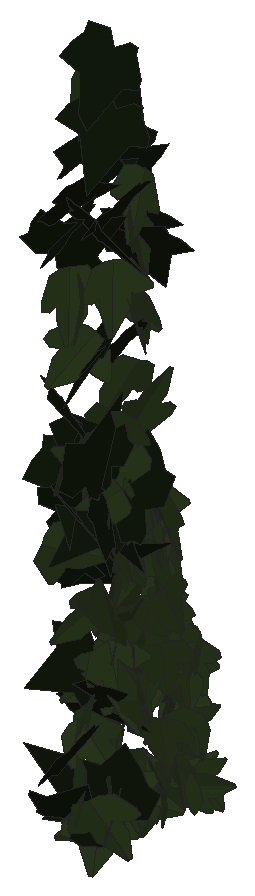
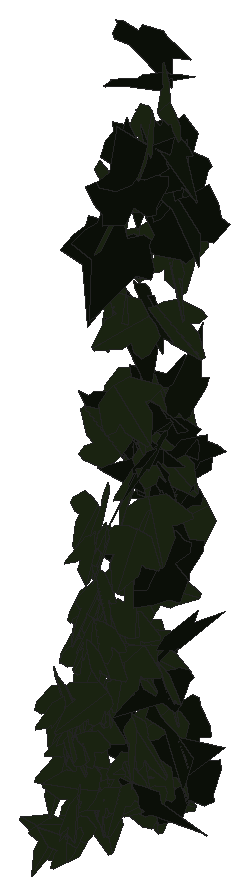
# SketchUp Ruby script. Lengths in inches.
U = 1.inch
M = Sketchup.active_model
def pt(a) = Geom::Point3d.new(a.map { |v| v * U })
def face(e, loops, mat)
  f = e.add_face(loops[0].map { |a| pt(a) })
  loops[1..].each { |l| e.add_face(l.map { |a| pt(a) }).erase! }
  f.material = f.back_material = mat if mat
  f
end
# faces: each face lists its corners as indices into pts; further lists are holes
def faces(e, pts, list, mat = nil) = list.each { |f| face(e, (f[0].is_a?(Array) ? f : [f]).map { |l| l.map { |i| pts[i] } }, mat) }
# xy, xz, yz: faces in a plane at the given z, y or x. An outline is a flat list of corners, or four numbers for a rectangle; further outlines are holes
def ring(l) = l.size == 4 ? [[l[0], l[1]], [l[2], l[1]], [l[2], l[3]], [l[0], l[3]]] : l.each_slice(2).to_a
def flat(e, list, mat, &to3) = list.each { |f| face(e, (f[0].is_a?(Array) ? f : [f]).map { |l| ring(l).map { |u, v| to3.(u, v) } }, mat) }
def xy(e, z, list, mat = nil) = flat(e, list, mat) { |x, y| [x, y, z] }
def xz(e, y, list, mat = nil) = flat(e, list, mat) { |x, z| [x, y, z] }
def yz(e, x, list, mat = nil) = flat(e, list, mat) { |y, z| [x, y, z] }
def lines(e, pts, list) = list.each { |a, b| e.add_line(pt(pts[a]), pt(pts[b])) }
# prism: a flat outline (further loops are holes) pulled along v
def prism(e, loops, v, mat = nil)
  f = face(e, loops, mat); d = Geom::Vector3d.new(v.map { |x| x * U })
  f.pushpull(f.normal.samedirection?(d) ? d.length : -d.length)
end
def box(e, o, s, mat = nil) = prism(e, [[o, [o[0] + s[0], o[1], o[2]], [o[0] + s[0], o[1] + s[1], o[2]], [o[0], o[1] + s[1], o[2]]]], [0, 0, s[2]], mat)
def at(x, y, z, deg = 0) = Geom::Transformation.translation(pt([x, y, z])) * Geom::Transformation.rotation(ORIGIN, Z_AXIS, deg.degrees)
def axes(o, x, y, z) = Geom::Transformation.new([*x, 0, *y, 0, *z, 0, *pt(o).to_a, 1])
def part(name) = M.definitions.add(name)
# library, detail: a bought-in or finely detailed component or shape, given as its bounding box
def library(name, o, s) = part(name).tap { |d| box(d.entities, o, s) }
def detail(e, o, s) = box(e.add_group.entities, o, s)
def put(e, d, t, mat = nil) = e.add_instance(d, t).tap { |i| i.material = mat if mat }
def group(e, t, mat = nil) = e.add_group.tap { |g| g.transformation = t; g.material = mat if mat }.entities
root = M.entities
M.materials.add("efeu1").color = [18, 25, 13]
M.materials.add("efeu2").color = [43, 57, 29]
c1 = part("ivyleaf_10")
p = [[0,0.5,-0.03],[-0.0625,2.02,-0.43],[-0.19,2.01,-0.46],[-0.54,1.05,-0.29],[-0.52,0.625,-0.18],[-0.83,0.76,-0.28],
  [-1.16,0.64,-0.33],[-1.15,0.33,-0.24],[-0.77,-0.39,0.02],[-0.3,-0.51,0.16],[0.04,-0.48,0.23],[-0.02,2.01,-0.4375],
  [-0.06,2.01,-0.43],[0.04,-0.49,0.23],[0.67,-0.49,0.14],[1.38,0.36,-0.2],[1.375,0.51,-0.24],[0.81,0.65,-0.19],
  [0.62,0.59,-0.15],[0.6,1.09,-0.28],[0.5,1.23,-0.31]]
faces(c1.entities,p,[[0,1,2,3,4,5,6,7,8,9,10],[11,12,0,13,14,15,16,17,18,19,20]],"efeu2")
c2 = part("ivyleaf_9")
p = [[1.54,2.16,1.25],[1.36,2.04,1.19],[-0.21,0.99,0.68],[-0.71,1.11,0.82],[-0.85,0.86,0.67],[-0.8,0.17,0.21],
  [-0.9,-0.01,0.1],[-0.67,-0.16,-0.02],[-0.08,-0.08,-0.05],[-0.03,-0.6,-0.4],[0.65,-0.88,-0.66],[0.83,-0.6,-0.49],
  [1.29,-0.42,-0.43],[1.8125,-0.07,-0.26],[1.21,0.44,0.15]]
faces(c2.entities,p,[[0,1,2,3,4,5,6,7,8,9,10,11,12,13,14]],"efeu1")
put(root,c1,axes([599.61,135.3125,199.58],[0.25459,0.74075,-0.09449],[-0.04378,-0.08485,-0.78316],[-0.74547,0.25796,0.01373]))
put(root,c2,axes([600.47,134.93,194.36],[-0.1452,-0.29097,0.75939],[0.47939,0.59249,0.31869],[-0.6569,0.4967,0.06471]))
put(root,c2,axes([599.87,135.34,201.62],[0.69033,-0.30203,0.29474],[0.27103,-0.11584,-0.7535],[0.32347,0.74162,0.00234]))
put(root,c2,axes([599.35,135.42,193.1],[0.66811,-0.36657,0.18485],[0.15857,-0.09525,-0.76204],[0.37868,0.68664,-0.00702]))
put(root,c2,axes([600.54,135.93,204.56],[-0.44801,-0.6677,-0.02671],[0.21926,-0.1165,-0.76525],[0.63124,-0.43342,0.24685]))
put(root,c2,axes([599.72,134.79,202.14],[0.33144,0.50901,0.52105],[0.21464,0.47879,-0.60426],[-0.69607,0.39001,0.06177]))
put(root,c1,axes([600.47,135.39,184.69],[-0.63533,-0.28347,-0.34153],[0.3443,0.06158,-0.6916],[0.2801,-0.71868,0.07545]))
put(root,c1,axes([600.65,135.61,189.94],[-0.75953,0.14608,0.00324],[-0.00226,-0.02889,0.77291],[0.1461,0.75899,0.0288]))
put(root,c2,axes([599.11,136.01,195.31],[0.65886,-0.48789,-0.17009],[0.13682,-0.10105,0.81984],[-0.49824,-0.67292,0.0002]))
put(root,c2,axes([600.57,135.81,193.25],[-0.76946,-0.09746,0.02751],[-0.02725,-0.00375,-0.77561],[0.09753,-0.76994,0.0003]))
put(root,c1,axes([599.98,135.22,194.75],[-0.14615,-0.59855,-0.50014],[0.09872,0.49056,-0.61592],[0.77373,-0.17565,-0.01589]))
put(root,c2,axes([599.76,135.14,201.15],[-0.24745,0.70178,0.28483],[-0.13987,0.25215,-0.74277],[-0.74435,-0.28068,0.04488]))
put(root,c1,axes([599.78,135.72,197.74],[0.64047,0.16565,-0.40422],[-0.38885,-0.11073,-0.66149],[-0.19908,0.74922,-0.00839]))
put(root,c2,axes([599.37,136.24,188.22],[-0.27899,-0.33499,0.62399],[-0.26309,-0.57365,-0.4256],[0.65755,-0.37166,0.09447]))
put(root,c2,axes([599.06,135.53,200.21],[-0.02269,-0.17555,0.78499],[0.79916,-0.09423,0.00203],[0.09148,0.77965,0.17699]))
put(root,c1,axes([599.81,135.41,199.17],[0.39893,-0.43032,-0.51826],[-0.29263,0.43181,-0.5838],[0.60674,0.4912,0.05918]))
put(root,c1,axes([599.63,135.63,185.125],[0.56093,-0.54131,-0.25315],[-0.16271,0.19574,-0.77907],[0.575,0.58345,0.0265]))
put(root,c2,axes([599,135.84,183.79],[0.81492,0.12743,-0.00059],[-0.00063,0.0079,0.82479],[0.12743,-0.81489,0.0079]))
put(root,c2,axes([600.53,135.44,193.51],[0.54513,-0.39287,-0.54286],[-0.41828,0.34724,-0.67132],[0.52353,0.6865,0.0289]))
put(root,c1,axes([600.56,135.71,193.61],[0.57359,-0.02819,-0.53938],[-0.53417,0.08681,-0.57259],[0.07992,0.78256,0.04409]))
put(root,c1,axes([599.17,135.3,191.875],[-0.18057,-0.24308,-0.707],[0.53832,0.46244,-0.29648],[0.51879,-0.56445,0.06157]))
put(root,c2,axes([599.26,135.39,192.91],[0.38302,0.07637,0.71638],[0.70633,0.12,-0.39043],[-0.1419,0.80343,-0.00978]))
put(root,c1,axes([600.06,136.16,194.84],[0.04642,-0.58409,0.4608],[0.17515,-0.44014,-0.57555],[0.72306,0.14411,0.10983]))
put(root,c2,axes([599.5625,135.36,186.07],[-0.08015,0.77152,0.09421],[0.00643,0.09537,-0.7755],[-0.77722,-0.07877,-0.01613]))
put(root,c2,axes([600.95,135.39,202.17],[-0.0345,0.77818,0.12393],[-0.02455,0.12292,-0.77872],[-0.78761,-0.03792,0.01884]))
put(root,c2,axes([600.18,136.16,198.08],[-0.57313,0.13169,-0.49289],[0.41392,-0.31333,-0.56503],[-0.29824,-0.68793,0.163]))
put(root,c1,axes([599.76,136.24,189.97],[0.11652,0.36173,-0.6354],[-0.38291,-0.51793,-0.36507],[-0.62286,0.38608,0.10557]))
put(root,c2,axes([599.22,136.17,194.06],[-0.29701,-0.75287,-0.19878],[0.07643,0.18354,-0.80933],[0.77491,-0.30667,0.00364]))
put(root,c1,axes([600.56,135.88,199.875],[0.31957,0.70205,-0.07493],[-0.04501,-0.06182,-0.77121],[-0.7046,0.32236,0.01528]))
put(root,c2,axes([600.27,136.18,206.11],[-0.70352,-0.30417,-0.2809],[0.25777,0.11162,-0.76646],[0.32401,-0.74926,-0.00015]))
put(root,c2,axes([600.6,135.67,194.61],[-0.19858,0.26734,0.70436],[-0.52025,0.47819,-0.32817],[-0.54491,-0.55398,0.05664]))
put(root,c1,axes([600.28,136.15,193.57],[-0.48343,0.19234,-0.52331],[0.37826,-0.3957,-0.49487],[-0.4096,-0.59244,0.16064]))
put(root,c1,axes([599.64,136.25,193.97],[-0.41697,-0.3947,0.51197],[-0.3114,-0.41126,-0.57067],[0.56651,-0.51657,0.06314]))
put(root,c2,axes([600.09,136.17,193.51],[-0.46393,-0.15637,-0.58102],[0.55507,0.17195,-0.48948],[0.23224,-0.72336,0.00925]))
put(root,c2,axes([600.65,136.05,184.31],[-0.14707,0.03827,1.04854],[-0.97388,0.38903,-0.1508],[-0.39045,-0.98475,-0.01882]))
put(root,c1,axes([600.08,136.55,184.39],[0.11062,-0.1787,0.75635],[0.50491,-0.56425,-0.20716],[0.59081,0.51567,0.03543]))
put(root,c2,axes([601.5625,135.77,193.66],[-0.38197,0.35338,0.93629],[-0.73703,0.5786,-0.51906],[-0.67698,-0.82931,0.03683]))
put(root,c1,axes([600.08,136.4375,183.72],[-0.0976,-0.13301,0.70046],[-0.43756,-0.54702,-0.16484],[0.56292,-0.44826,-0.00668]))
put(root,c1,axes([599.45,136.2,187.38],[0.5612,-0.46532,-0.04269],[-0.03201,0.02827,-0.72901],[0.46617,0.56211,0.00133]))
put(root,c1,axes([600.64,135.9375,192.8],[-0.23885,0.72018,0.10211],[-0.03067,0.09741,-0.75875],[-0.72674,-0.24081,-0.00154]))
put(root,c1,axes([600.84,136.16,194.79],[0.6312,-0.02327,-0.4378],[-0.4351,0.06103,-0.63055],[0.05386,0.76574,0.03695]))
put(root,c1,axes([599.83,136.18,183.93],[0.66606,0.36568,-0.02318],[-0.0279,0.00266,-0.75968],[-0.36535,0.66646,0.01575]))
put(root,c1,axes([600.47,136.08,195.6],[-0.77075,-0.02347,0.01456],[-0.01444,-0.00393,-0.7711],[0.02354,-0.77088,0.00349]))
put(root,c1,axes([599.99,136.45,188.09],[0.37902,0.21791,-0.56361],[-0.48948,-0.2794,-0.43719],[-0.35432,0.61906,0.00107]))
put(root,c2,axes([599.4,136.21,194.93],[-0.27111,-0.32834,-0.63014],[0.4292,0.46183,-0.4253],[0.56627,-0.50723,0.02066]))
put(root,c2,axes([599.74,135.96,203.34],[-0.35726,0.66482,0.19347],[-0.19013,0.11515,-0.74675],[-0.66578,-0.38962,0.10943]))
put(root,c1,axes([599.45,136.15,186.23],[0.53121,0.17237,0.52143],[0.47237,0.2266,-0.55615],[-0.28011,0.70903,0.05098]))
put(root,c2,axes([599.51,135.91,187.47],[0.69986,0.25095,0.17026],[0.15858,0.06216,-0.74347],[-0.25849,0.71758,0.00486]))
put(root,c1,axes([598.93,136.6,204.65],[0.38824,-0.24458,0.67301],[0.62417,-0.25963,-0.45442],[0.35097,0.7323,0.06367]))
put(root,c2,axes([599.21,136.44,190.71],[0.46157,0.47025,0.48001],[-0.40032,-0.2753,0.65464],[0.53972,-0.60636,0.07504]))
put(root,c2,axes([600.46,136.06,197.83],[-0.10274,0.75967,-0.0663],[-0.00772,-0.06794,-0.7664],[-0.76252,-0.10167,0.01669]))
put(root,c1,axes([600.84,136.26,187.6],[-0.24765,0.06834,0.70542],[-0.70865,-0.01368,-0.24746],[-0.00967,-0.7475,0.06903]))
put(root,c2,axes([599.52,136.25,194.48],[0.57557,-0.35458,-0.36575],[-0.29442,0.21882,-0.67544],[0.41572,0.64589,0.02804]))
put(root,c1,axes([600.07,136.54,187.75],[0.44674,-0.00697,0.55607],[0.55599,-0.00955,-0.4468],[0.01181,0.71323,-0.00055]))
put(root,c1,axes([600.1,136.38,188.55],[0.30828,0.63854,0.09708],[0.04081,0.08809,-0.70906],[-0.64459,0.31097,0.00154]))
put(root,c1,axes([599.84,136.4,184.51],[-0.49715,-0.34902,-0.37461],[0.34351,0.15982,-0.60478],[0.37966,-0.60162,0.05667]))
put(root,c1,axes([600.77,136.39,198.85],[-0.49328,0.55088,0.22236],[-0.14824,0.16573,-0.73945],[-0.57527,-0.51507,-0.00012]))
put(root,c1,axes([599.49,136.74,192.43],[-0.5124,-0.51644,0.16325],[-0.11,-0.12083,-0.72747],[0.53034,-0.52403,0.00685]))
put(root,c2,axes([599.11,136.36,190.88],[0.29878,0.58881,-0.48771],[0.22699,0.4317,0.66025],[0.73009,-0.37518,-0.00569]))
put(root,c1,axes([599.88,137.27,188.83],[0.01403,-0.49345,-0.52699],[0.08326,-0.52246,0.49143],[-0.71713,-0.07031,0.04675]))
put(root,c1,axes([599.73,136.62,192.06],[-0.34414,0.61957,0.16459],[-0.09892,0.13325,-0.70842],[-0.63338,-0.35745,0.02121]))
put(root,c1,axes([600.46,137.02,202],[0.75126,-0.22701,0.09119],[0.08533,-0.03284,-0.78478],[0.22927,0.75606,-0.00671]))
put(root,c1,axes([599.6875,137.19,189.3],[-0.01932,-0.70925,-0.29727],[-0.01108,-0.29708,0.70951],[-0.76895,0.02211,-0.00276]))
put(root,c2,axes([599.82,137.13,184.1],[-0.677,0.07178,0.336],[-0.33761,-0.00112,-0.68],[-0.0638,-0.75579,0.03292]))
put(root,c1,axes([599.88,136.82,185.71],[-0.23043,0.16344,0.66486],[-0.67726,0.04838,-0.24662],[-0.10032,-0.70199,0.1378]))
put(root,c1,axes([599.78,136.85,183.73],[0.566,0.39545,-0.18804],[0.15171,0.11118,0.69045],[0.41077,-0.58596,0.0041]))
put(root,c1,axes([600.25,136.68,191.5],[-0.17568,0.58332,0.39693],[-0.13325,0.37426,-0.60898],[-0.69286,-0.21988,0.01648]))
put(root,c1,axes([599.37,137.05,204.11],[-0.62281,0.48346,0.04788],[-0.07678,-0.02108,-0.78586],[-0.47972,-0.62429,0.06362]))
put(root,c1,axes([600.33,137.11,200.91],[-0.23561,0.74297,-0.0561],[0.00333,-0.05779,-0.7793],[-0.74508,-0.2352,0.01426]))
put(root,c1,axes([599.9375,137.44,190.98],[0.07035,0.59572,-0.35334],[-0.12506,-0.33839,-0.59543],[-0.68124,0.12364,0.07282]))
put(root,c1,axes([600.17,137.01,184.29],[-0.14812,-0.20858,-0.64289],[0.60862,0.24504,-0.21972],[0.29391,-0.61253,0.13101]))
put(root,c1,axes([600.33,137.16,198.73],[-0.67344,0.31601,0.08048],[-0.08674,0.00442,-0.74318],[-0.31435,-0.67822,0.03266]))
put(root,c2,axes([599.53,137.42,201.84],[0.50269,0.42833,0.39648],[-0.32958,-0.22353,0.65937],[0.4817,-0.59994,0.03739]))
put(root,c1,axes([599.92,136.92,185.63],[-0.11854,0.3022,0.62893],[-0.49713,0.41107,-0.29122],[-0.48963,-0.49053,0.14342]))
put(root,c1,axes([599.71,137.65,196.11],[-0.27798,-0.59908,0.34965],[-0.1361,-0.32226,-0.66035],[0.68017,-0.30932,0.01077]))
put(root,c1,axes([599.52,137.2,188.37],[0.19237,0.64879,0.20005],[0.05394,0.19266,-0.67671],[-0.67679,0.19976,0.00293]))
put(root,c1,axes([599.89,137.11,184.86],[-0.13917,-0.49336,-0.45798],[0.11662,0.44292,-0.51257],[0.66298,-0.18147,-0.00598]))
put(root,c1,axes([599.84,137.41,189.24],[-0.43087,-0.5345,-0.05392],[0.03694,0.03947,-0.68653],[0.53594,-0.43243,0.00398]))
put(root,c2,axes([600.3,137.1875,200.33],[0.57196,0.49681,-0.19291],[-0.12996,-0.14442,-0.75725],[-0.51686,0.58609,-0.02307]))
put(root,c2,axes([599.57,137.23,202.59],[-0.40035,-0.31504,0.58593],[0.46008,0.36282,0.50944],[-0.48051,0.60988,-0.0004]))
put(root,c1,axes([600.1875,137.39,187.63],[-0.2879,0.61659,0.02274],[-0.00736,0.02166,-0.68049],[-0.61697,-0.28798,-0.00249]))
put(root,c1,axes([600.82,137.52,188.43],[-0.4748,-0.51111,-0.06286],[0.03787,0.05062,-0.69758],[0.51356,-0.47626,-0.00668]))
put(root,c1,axes([599.37,137.36,198.375],[0.45942,0.00439,0.59474],[0.50578,0.39251,-0.3936],[-0.31292,0.64087,0.23699]))
put(root,c1,axes([600.97,137.26,184.62],[0.23805,-0.0913,-0.66321],[-0.37568,0.5644,-0.21254],[0.55412,0.42187,0.14082]))
put(root,c1,axes([600.2,137.13,188.67],[0.16467,0.00962,-0.6977],[-0.12685,0.70533,-0.02021],[0.68614,0.12809,0.1637]))
put(root,c1,axes([599.63,137.61,188.4375],[-0.52654,-0.46657,-0.10247],[0.07665,0.068,-0.70351],[0.4715,-0.53209,-0.00006]))
put(root,c1,axes([600.29,137.84,184.02],[-0.44214,-0.50523,0.15799],[-0.10416,-0.1188,-0.67137],[0.519,-0.45425,-0.00014]))
put(root,c1,axes([600.68,137.7,186.15],[-0.62839,-0.25885,0.01291],[-0.01416,0.00048,-0.67959],[0.25879,-0.62852,-0.00584]))
put(root,c1,axes([600.05,137.81,184.59],[0.19149,0.62767,-0.13612],[-0.06241,-0.12319,-0.65581],[-0.63922,0.20006,0.02325]))
put(root,c1,axes([600.61,137.8125,192.48],[-0.56144,0.32969,-0.26763],[0.20912,-0.17147,-0.64993],[-0.36959,-0.59787,0.03882]))
put(root,c2,axes([599.76,137.46,200.67],[0.59397,0.46252,-0.12405],[-0.08179,-0.09676,-0.75237],[-0.47183,0.59902,-0.02574]))
put(root,c1,axes([600.45,137.41,187.01],[0.32305,0.00931,0.61207],[-0.47972,0.43375,0.24659],[-0.38025,-0.53931,0.2089]))
put(root,c1,axes([600.56,137.77,184.43],[0.39815,-0.4127,-0.34597],[-0.21502,0.27265,-0.57269],[0.49375,0.45153,0.02958]))
put(root,c1,axes([599.26,137.8125,192.09],[-0.68969,-0.11486,-0.10799],[0.10527,0.02523,-0.69914],[0.11736,-0.69763,-0.00751]))
put(root,c1,axes([600.68,137.95,184.87],[0.45415,-0.49626,-0.11124],[-0.07698,0.08034,-0.6727],[0.50272,0.46062,-0.00251]))
put(root,c1,axes([599.7,137.85,184.46],[0.24781,0.62315,0.07576],[0.02737,0.07065,-0.67062],[-0.62715,0.24931,0.00067]))
put(root,c1,axes([599.94,137.92,187.6],[0.38119,0.55348,0.0293],[0.01601,0.02456,-0.67204],[-0.55402,0.38153,0.00075]))
put(root,c1,axes([600.68,137.83,189.86],[-0.02735,-0.64301,-0.28223],[0.16338,0.26887,-0.6284],[0.68296,-0.09007,0.13903]))
put(root,c1,axes([599.92,137.79,194.74],[-0.07633,-0.65052,0.34299],[0.02698,0.34212,0.65488],[-0.7349,0.08013,-0.01158]))
put(root,c1,axes([599.9,138.16,193.18],[-0.33641,0.64415,-0.04422],[-0.01433,-0.0573,-0.72565],[-0.64551,-0.33443,0.03915]))
put(root,c1,axes([599.78,138.3125,192.01],[-0.34303,0.57342,-0.25785],[0.12338,-0.22662,-0.66812],[-0.6165,-0.36442,0.00976]))
put(root,c1,axes([600.05,138.32,192.08],[0.05771,0.70095,0.01442],[0.0025,0.01426,-0.70332],[-0.7011,0.05775,-0.00132]))
put(root,c1,axes([599.84,138.46,191.14],[0.58489,-0.38305,-0.11515],[-0.06762,0.10636,-0.69728],[0.39423,0.58655,0.05124]))
put(root,c1,axes([600.49,138.29,185.95],[-0.45004,-0.36453,-0.3079],[0.23093,0.20398,-0.57904],[0.41756,-0.5057,-0.01161]))
put(root,c1,axes([600.05,138.84,188.76],[-0.1915,0.5091,0.4197],[0.14854,-0.39254,0.54393],[0.64286,0.24236,-0.00065]))
put(root,c1,axes([599.9,138.59,189.84],[-0.24333,0.63919,-0.06217],[0.01193,-0.06197,-0.68385],[-0.6421,-0.24338,0.01085]))
put(root,c1,axes([599.79,138.63,188.93],[-0.63082,-0.25518,-0.17458],[0.18606,0.00349,-0.67742],[0.24693,-0.65452,0.06445]))
put(root,c1,axes([599.87,138.66,187.82],[-0.6264,0.27097,-0.10557],[0.06699,-0.10952,-0.67857],[-0.28299,-0.62572,0.07305]))
put(root,c1,axes([599.59,138.77,189.84],[0.68137,-0.00889,0.07959],[0.07961,0.00142,-0.68142],[0.00866,0.686,0.00244]))
put(root,c1,axes([599.79,138.88,189.28],[0.59755,-0.29129,0.15191],[0.14123,-0.05691,-0.66468],[0.29661,0.61392,0.01046]))
put(root,c1,axes([599.97,138.97,186.1875],[0.19472,-0.63629,-0.13979],[0.0386,-0.13438,0.66541],[-0.65032,-0.19849,-0.00237]))
put(root,c1,axes([599.97,138.51,190.6],[-0.20746,0.53421,0.39539],[-0.13551,0.3715,-0.57304],[-0.65065,-0.2477,-0.00672]))
put(root,c1,axes([600.13,139.08,186.77],[0.23909,-0.6235,0.08478],[0.03837,-0.07607,-0.66771],[0.62806,0.242,0.00853]))
put(root,c1,axes([600.59,139.07,187.93],[0.52235,-0.42194,-0.0248],[-0.01929,0.01557,-0.67148],[0.42223,0.5227,-0.00001]))
put(root,c1,axes([600.02,139.03,186.43],[0.4668,0.46114,-0.07733],[-0.0641,-0.04513,-0.65604],[-0.46316,0.471,0.01286]))
put(root,c1,axes([600.52,139.02,187.35],[0.08791,0.65998,-0.05919],[-0.07771,-0.04903,-0.66209],[-0.65806,0.09396,0.07028]))
put(root,c1,axes([600.15,138.96,187.03],[-0.18248,0.65464,0.02724],[-0.00683,0.02637,-0.6796],[-0.65518,-0.18261,-0.0005]))
put(root,c1,axes([600.4,139.01,187.57],[-0.48886,-0.41605,-0.19531],[0.18222,0.08632,-0.63997],[0.42195,-0.5193,0.0501]))
put(root,c1,axes([600.05,139.11,184.47],[-0.20501,0.60664,-0.15783],[0.06077,-0.14605,-0.64026],[-0.62389,-0.21357,-0.0105]))
put(root,c1,axes([599.89,138.93,185.03],[0.02505,-0.31048,0.60151],[0.05548,0.60084,0.30782],[-0.67464,0.03789,0.04765]))
put(root,c1,axes([600.22,139.32,183.56],[-0.16993,-0.16801,0.60796],[0.55671,0.25603,0.22636],[-0.29651,0.57701,0.07658]))
put(root,c1,axes([600.48,139.2,185.58],[0.00451,0.60743,0.24342],[-0.15185,0.23775,-0.59047],[-0.63652,-0.05242,0.14259]))
put(root,c1,axes([599.79,139.49,184.88],[-0.19155,0.60654,-0.11976],[-0.04593,-0.13899,-0.63047],[-0.61654,-0.17809,0.08418]))
put(root,c1,axes([600,139.11,183.55],[0.2031,0.25998,-0.56722],[0.35181,0.44494,0.3299],[0.51533,-0.40622,-0.00167]))
put(root,c1,axes([599.26,139.27,188.07],[0.14568,0.33378,0.55382],[0.16186,0.5308,-0.36249],[-0.62604,0.21491,0.03515]))
put(root,c1,axes([600.49,139.39,183.8125],[0.02396,0.51162,0.38768],[-0.03834,0.3884,-0.5102],[-0.64077,-0.00411,0.04503]))
